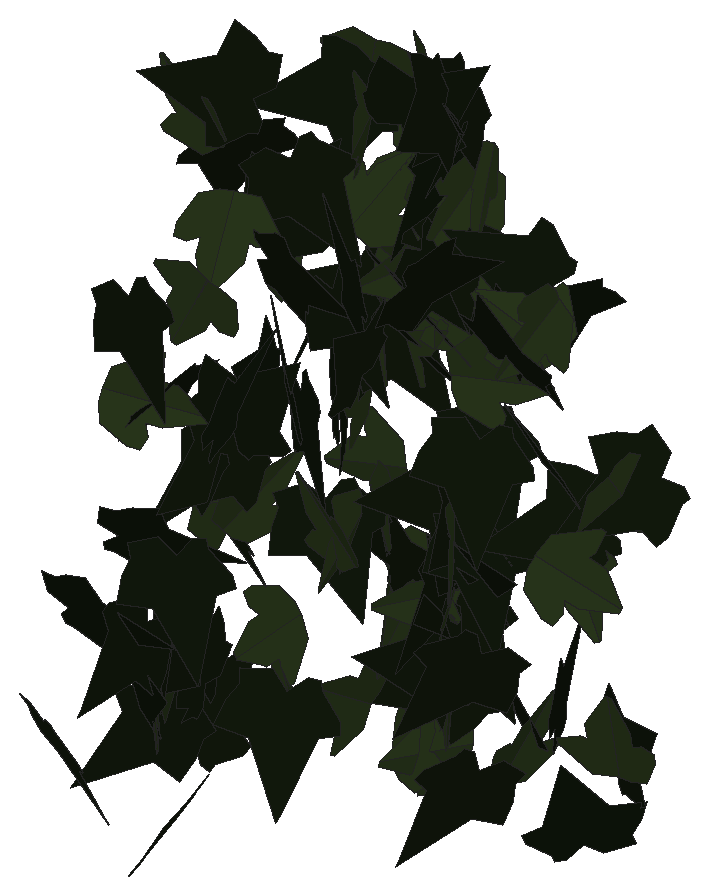
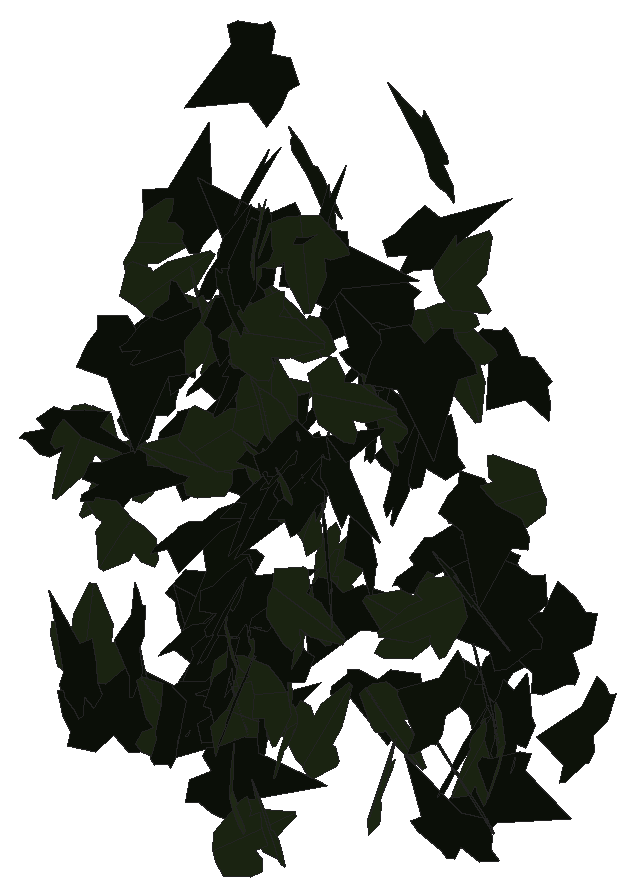
# SketchUp Ruby script. Lengths in inches.
U = 1.inch
M = Sketchup.active_model
def pt(a) = Geom::Point3d.new(a.map { |v| v * U })
def face(e, loops, mat)
  f = e.add_face(loops[0].map { |a| pt(a) })
  loops[1..].each { |l| e.add_face(l.map { |a| pt(a) }).erase! }
  f.material = f.back_material = mat if mat
  f
end
# faces: each face lists its corners as indices into pts; further lists are holes
def faces(e, pts, list, mat = nil) = list.each { |f| face(e, (f[0].is_a?(Array) ? f : [f]).map { |l| l.map { |i| pts[i] } }, mat) }
# xy, xz, yz: faces in a plane at the given z, y or x. An outline is a flat list of corners, or four numbers for a rectangle; further outlines are holes
def ring(l) = l.size == 4 ? [[l[0], l[1]], [l[2], l[1]], [l[2], l[3]], [l[0], l[3]]] : l.each_slice(2).to_a
def flat(e, list, mat, &to3) = list.each { |f| face(e, (f[0].is_a?(Array) ? f : [f]).map { |l| ring(l).map { |u, v| to3.(u, v) } }, mat) }
def xy(e, z, list, mat = nil) = flat(e, list, mat) { |x, y| [x, y, z] }
def xz(e, y, list, mat = nil) = flat(e, list, mat) { |x, z| [x, y, z] }
def yz(e, x, list, mat = nil) = flat(e, list, mat) { |y, z| [x, y, z] }
def lines(e, pts, list) = list.each { |a, b| e.add_line(pt(pts[a]), pt(pts[b])) }
# prism: a flat outline (further loops are holes) pulled along v
def prism(e, loops, v, mat = nil)
  f = face(e, loops, mat); d = Geom::Vector3d.new(v.map { |x| x * U })
  f.pushpull(f.normal.samedirection?(d) ? d.length : -d.length)
end
def box(e, o, s, mat = nil) = prism(e, [[o, [o[0] + s[0], o[1], o[2]], [o[0] + s[0], o[1] + s[1], o[2]], [o[0], o[1] + s[1], o[2]]]], [0, 0, s[2]], mat)
def at(x, y, z, deg = 0) = Geom::Transformation.translation(pt([x, y, z])) * Geom::Transformation.rotation(ORIGIN, Z_AXIS, deg.degrees)
def axes(o, x, y, z) = Geom::Transformation.new([*x, 0, *y, 0, *z, 0, *pt(o).to_a, 1])
def part(name) = M.definitions.add(name)
# library, detail: a bought-in or finely detailed component or shape, given as its bounding box
def library(name, o, s) = part(name).tap { |d| box(d.entities, o, s) }
def detail(e, o, s) = box(e.add_group.entities, o, s)
def put(e, d, t, mat = nil) = e.add_instance(d, t).tap { |i| i.material = mat if mat }
def group(e, t, mat = nil) = e.add_group.tap { |g| g.transformation = t; g.material = mat if mat }.entities
root = M.entities
M.materials.add("efeu1").color = [18, 25, 13]
M.materials.add("efeu2").color = [43, 57, 29]
c1 = part("ivyleaf_9")
p = [[1.54,2.16,1.25],[1.36,2.04,1.19],[-0.21,0.99,0.68],[-0.71,1.11,0.82],[-0.85,0.86,0.67],[-0.8,0.17,0.21],
  [-0.9,-0.01,0.1],[-0.67,-0.16,-0.02],[-0.08,-0.08,-0.05],[-0.03,-0.6,-0.4],[0.65,-0.88,-0.66],[0.83,-0.6,-0.49],
  [1.29,-0.42,-0.43],[1.8125,-0.07,-0.26],[1.21,0.44,0.15]]
faces(c1.entities,p,[[0,1,2,3,4,5,6,7,8,9,10,11,12,13,14]],"efeu1")
c2 = part("ivyleaf_10")
p = [[0,0.5,-0.03],[-0.0625,2.02,-0.43],[-0.19,2.01,-0.46],[-0.54,1.05,-0.29],[-0.52,0.625,-0.18],[-0.83,0.76,-0.28],
  [-1.16,0.64,-0.33],[-1.15,0.33,-0.24],[-0.77,-0.39,0.02],[-0.3,-0.51,0.16],[0.04,-0.48,0.23],[-0.02,2.01,-0.4375],
  [-0.06,2.01,-0.43],[0.04,-0.49,0.23],[0.67,-0.49,0.14],[1.38,0.36,-0.2],[1.375,0.51,-0.24],[0.81,0.65,-0.19],
  [0.62,0.59,-0.15],[0.6,1.09,-0.28],[0.5,1.23,-0.31]]
faces(c2.entities,p,[[0,1,2,3,4,5,6,7,8,9,10],[11,12,0,13,14,15,16,17,18,19,20]],"efeu2")
put(root,c1,axes([47.99,215.16,220.86],[-0.17169,0.44086,0.16175],[0.0482,-0.15477,0.47299],[0.46712,0.17801,0.01065]))
put(root,c1,axes([46.04,216.63,214.23],[-0.07459,0.45103,0.20252],[-0.03957,0.1987,-0.45711],[-0.49282,-0.08422,0.00606]))
put(root,c1,axes([43.89,217.16,214.625],[0.30514,-0.33363,0.2135],[0.14379,-0.15781,-0.45213],[0.36907,0.33732,-0.00036]))
put(root,c1,axes([48.8,216.82,221.22],[-0.16626,0.34154,0.32513],[-0.13737,0.29472,-0.37983],[-0.4511,-0.21563,-0.00417]))
put(root,c1,axes([49.54,216.83,222.625],[-0.06882,0.21369,-0.44676],[-0.12086,0.43017,0.22438],[0.48027,0.13888,-0.00756]))
put(root,c1,axes([44.74,217.89,215.97],[0.05227,-0.05863,-0.49379],[0.24772,-0.42744,0.07698],[-0.43116,-0.25269,-0.01564]))
put(root,c1,axes([43.93,217.58,216.05],[0.28747,-0.12982,0.38796],[0.36207,-0.13998,-0.31513],[0.19043,0.46212,0.01353]))
put(root,c1,axes([49.72,217.85,217.31],[0.00747,0.18447,-0.46467],[-0.07922,-0.45841,-0.18326],[-0.49363,0.07636,0.02238]))
put(root,c1,axes([45.33,217.75,217.09],[-0.26087,-0.25582,-0.34133],[0.23496,0.24775,-0.36526],[0.35601,-0.35096,-0.00905]))
put(root,c1,axes([44.6,217.78,220.27],[-0.21419,-0.0866,-0.44342],[0.40773,0.17435,-0.231],[0.19463,-0.46055,-0.00407]))
put(root,c1,axes([49.43,218.17,215.51],[-0.02735,0.20302,-0.45611],[0.02463,-0.45569,-0.20431],[-0.49864,-0.03364,0.01493]))
put(root,c1,axes([44.26,218.28,214.91],[0.06762,-0.11488,0.4819],[0.22476,-0.42632,-0.13317],[0.44149,0.23463,-0.00601]))
put(root,c1,axes([47.65,218.22,221.05],[0.10012,-0.38158,0.3072],[-0.02038,0.31004,0.39174],[-0.48945,-0.09096,0.04653]))
put(root,c2,axes([45.28,218.3,220.42],[-0.42148,-0.06864,0.26009],[-0.25219,-0.06735,-0.42645],[0.09358,-0.49066,0.02216]))
put(root,c2,axes([44.33,218.53,214.92],[-0.15127,0.27122,-0.39186],[0.1831,-0.3465,-0.3105],[-0.43999,-0.23744,0.00551]))
put(root,c1,axes([44.46,218.74,214.35],[-0.02016,0.00124,-0.49959],[0.01647,-0.49973,-0.0019],[-0.49932,-0.01653,0.02011]))
put(root,c1,axes([44.12,218.28,216.77],[0.35731,-0.00643,0.3497],[0.34938,0.02964,-0.35644],[-0.01615,0.49908,0.02567]))
put(root,c1,axes([46.25,218.625,215.23],[-0.29745,-0.33879,-0.2162],[0.14429,0.16101,-0.45084],[0.3751,-0.3306,0.00198]))
put(root,c1,axes([45.59,218.51,218.67],[-0.16318,0.01348,0.47243],[0.40966,-0.2452,0.1485],[0.23569,0.43554,0.06898]))
put(root,c1,axes([49.5,218.69,220.84],[0.43274,-0.21487,0.12871],[-0.1132,0.0614,0.48313],[-0.22343,-0.44728,0.0045]))
put(root,c2,axes([44.12,218.29,218.62],[0.09254,0.11107,0.47864],[0.27138,0.39448,-0.14401],[-0.40962,0.28644,0.01272]))
put(root,c1,axes([44.42,218.78,216.05],[-0.20659,-0.00926,-0.45523],[0.44787,-0.09422,-0.20134],[-0.08205,-0.49096,0.04722]))
put(root,c1,axes([46.41,218.61,218.98],[0.03367,-0.24189,0.4363],[-0.08064,0.4289,0.24401],[-0.4923,-0.0868,-0.01013]))
put(root,c2,axes([45.16,218.91,221.15],[0.36505,0.32327,-0.11059],[-0.0819,-0.07433,-0.48761],[-0.33171,0.37413,-0.00131]))
put(root,c1,axes([45.8,218.9375,220.72],[0.2344,0.04973,-0.43884],[0.42362,0.11519,0.23932],[0.12491,-0.484,0.01187]))
put(root,c1,axes([44.37,218.63,218.53],[0.02948,0.49035,0.09323],[0.00081,0.09335,-0.49121],[-0.49913,0.02911,0.00471]))
put(root,c1,axes([44.97,219.4,217.79],[-0.18945,-0.33461,0.3196],[-0.16866,-0.27166,-0.38439],[0.43089,-0.25345,-0.00994]))
put(root,c1,axes([44.76,219.12,217.71],[-0.46066,0.16849,-0.09697],[0.08681,-0.04487,-0.49036],[-0.17394,-0.46861,0.01209]))
put(root,c1,axes([44.34,219.44,215],[-0.02739,-0.2858,0.40935],[-0.0486,-0.40649,-0.28706],[0.49688,-0.05552,-0.00551]))
put(root,c2,axes([44.49,218.7,214.85],[-0.00152,-0.08865,-0.49208],[-0.04087,0.49045,-0.08823],[0.49832,0.03995,-0.00874]))
put(root,c2,axes([44.68,219.07,222.01],[-0.38714,0.10727,-0.29769],[-0.28541,0.08472,0.4017],[0.13662,0.48095,-0.00437]))
put(root,c1,axes([45.35,219.42,218.61],[-0.03353,0.0613,0.49509],[-0.10617,-0.48572,0.05295],[0.48745,-0.10157,0.04559]))
put(root,c1,axes([45.05,219.43,222.43],[-0.15128,0.00179,0.47656],[-0.39667,-0.2776,-0.12488],[0.26414,-0.41586,0.08541]))
put(root,c2,axes([49.49,219.46,221.06],[0.0773,0.22623,-0.43914],[-0.11682,-0.4235,-0.23874],[-0.47998,0.13951,-0.01262]))
put(root,c1,axes([46.31,219.43,218.86],[-0.0575,0.149,0.47381],[0.07117,-0.46958,0.1563],[0.49156,0.08542,0.03279]))
put(root,c1,axes([44.69,219.04,214.7],[-0.2061,0.29988,0.34292],[-0.19811,0.27993,-0.36386],[-0.41022,-0.28585,0.00343]))
put(root,c2,axes([46.54,219.27,217.01],[-0.35888,0.19083,-0.29118],[-0.27946,0.09148,0.40439],[0.20762,0.453,0.041]))
put(root,c1,axes([48.37,219.55,218.92],[-0.14024,-0.46394,-0.12286],[0.04991,0.1132,-0.48445],[0.47733,-0.14815,0.01456]))
put(root,c1,axes([44.375,219.3,213.77],[-0.28637,0.15636,0.37887],[0.33335,-0.18007,0.32627],[0.23848,0.43946,-0.00111]))
put(root,c2,axes([44.75,219.1,217.11],[-0.03995,-0.08244,-0.49154],[0.27053,0.41056,-0.09085],[0.41859,-0.2732,0.0118]))
put(root,c2,axes([46.43,219.84,214.7],[-0.05422,-0.25576,-0.4262],[-0.10347,-0.41353,0.26132],[-0.48616,0.11653,-0.00808]))
put(root,c2,axes([45.51,219.52,215.57],[0.3507,-0.14006,-0.32771],[-0.31087,0.10461,-0.37738],[0.17428,0.46844,-0.01371]))
put(root,c2,axes([46.23,219.89,216.98],[0.06099,-0.17211,0.46547],[0.21407,-0.41397,-0.18112],[0.44772,0.22138,0.02319]))
put(root,c1,axes([45.6875,219.46,221.76],[-0.1147,-0.20196,-0.44278],[0.21685,0.38605,-0.23226],[0.43568,-0.24531,-0.00097]))
put(root,c2,axes([49.13,219.76,220.46],[0.18596,0.30213,0.35233],[-0.20413,-0.28764,0.35439],[0.41683,-0.27565,0.01637]))
put(root,c1,axes([46.16,219.65,220.1],[0.22341,-0.41117,-0.17616],[-0.05671,0.16928,-0.46704],[0.4437,0.22866,0.029]))
put(root,c2,axes([44.96,219.41,216.84],[-0.0438,-0.33988,0.36409],[0.03814,0.36213,0.34265],[-0.49662,0.05779,-0.0058]))
put(root,c1,axes([48.92,219.9375,218.91],[0.40702,-0.15845,-0.24337],[0.2273,-0.08699,0.43677],[-0.18076,-0.46618,0.00122]))
put(root,c1,axes([45.46,219.92,218.35],[-0.1148,0.01134,-0.48651],[0.48636,-0.01439,-0.1151],[-0.01662,-0.49966,-0.00772]))
put(root,c1,axes([45.26,219.72,220.66],[-0.25055,0.15868,0.40255],[0.34038,-0.21491,0.29657],[0.26714,0.42265,-0.00034]))
put(root,c2,axes([49.52,219.5,217.7],[0.12167,0.28036,0.39572],[0.14907,0.36661,-0.30557],[-0.46149,0.19234,0.00563]))
put(root,c1,axes([45.91,219.81,217.15],[-0.18585,-0.3015,-0.35293],[0.1696,0.30978,-0.35394],[0.43208,-0.25127,-0.01287]))
put(root,c1,axes([49.61,219.95,213.91],[0.3522,0.14995,0.32167],[-0.29593,-0.12609,0.38279],[0.19591,-0.46002,-0.00007]))
put(root,c2,axes([45.31,219.84,214.26],[-0.26282,0.42147,-0.05736],[-0.03543,0.0455,0.49666],[0.42388,0.26513,0.00595]))
put(root,c1,axes([47.23,220.3125,222.67],[-0.04162,-0.23336,0.44024],[-0.06095,-0.43607,-0.23691],[0.49452,-0.07339,0.00786]))
put(root,c2,axes([46.13,220.22,222.125],[-0.07635,0.06216,0.49021],[0.33725,-0.35598,0.09767],[0.36115,0.34556,0.01243]))
put(root,c1,axes([48.32,220.09,220.36],[0.08806,0.0112,-0.49206],[0.48948,0.05033,0.08874],[0.05152,-0.49733,-0.0021]))
put(root,c1,axes([43.93,220.2,216.26],[0.22128,-0.33793,0.29468],[0.19915,-0.22035,-0.40223],[0.40172,0.29538,0.03708]))
put(root,c2,axes([45.25,219.86,220.04],[0.22068,0.00089,0.44867],[-0.43181,0.13621,0.21211],[-0.12185,-0.48109,0.06088]))
put(root,c2,axes([46.03,220.43,218.46],[-0.00525,-0.19823,-0.45899],[0.02373,-0.4586,0.19779],[-0.49941,-0.01971,0.01423]))
put(root,c2,axes([49.91,220.16,214.96],[-0.48711,-0.11174,-0.0153],[-0.01208,-0.01575,0.49961],[-0.11213,0.4871,0.01265]))
put(root,c1,axes([44.43,219.96,221.44],[0.13293,0.4408,-0.19501],[-0.06511,-0.18401,-0.46033],[-0.47759,0.14778,0.00848]))
put(root,c1,axes([49.42,220.41,217.86],[-0.30264,-0.14157,0.37198],[-0.31304,-0.20391,-0.3323],[0.24579,-0.43403,0.03479]))
put(root,c1,axes([45.96,220.46,222.43],[-0.10597,-0.16668,-0.45933],[-0.21301,-0.40725,0.19692],[-0.43977,0.23742,0.0153]))
put(root,c2,axes([46.19,220.16,220.98],[0.41876,-0.00156,-0.27319],[0.27284,0.02802,0.41806],[0.01401,-0.49921,0.02432]))
put(root,c2,axes([48.42,220.14,214.4],[0.03137,-0.45907,0.19564],[0.01505,0.1968,0.45939],[-0.49879,-0.02293,0.02617]))
put(root,c2,axes([46.08,220.5,219.41],[0.16434,-0.08747,0.46405],[0.39857,-0.23781,-0.18598],[0.25325,0.43104,-0.00844]))
put(root,c2,axes([46.08,220.54,217],[-0.06596,0.08423,-0.48842],[0.2724,-0.40548,-0.10671],[-0.41407,-0.28016,0.0076]))
put(root,c1,axes([49.16,220,215.32],[-0.00316,-0.01195,0.49985],[0.05719,0.49657,0.01224],[-0.49671,0.05725,-0.00177]))
put(root,c2,axes([49.0625,220.34,217.31],[0.41107,0.06457,0.27722],[0.27293,0.04886,-0.41608],[-0.08082,0.4934,0.00493]))
put(root,c1,axes([47.04,220.2,220.6875],[0.22053,-0.26657,-0.36098],[-0.20999,0.29415,-0.34551],[0.39658,0.30399,0.01778]))
put(root,c1,axes([47.14,220.72,214.99],[-0.10074,-0.06541,0.48536],[-0.38447,-0.29638,-0.11974],[0.30337,-0.39734,0.00942]))
put(root,c1,axes([49.63,220.57,214.75],[-0.03926,0.05589,0.49531],[0.23831,-0.43428,0.0679],[0.4378,0.24141,0.00746]))
put(root,c1,axes([50.08,220.6875,218.56],[-0.39718,-0.21572,0.21381],[-0.18545,-0.10651,-0.45196],[0.24054,-0.43832,0.00459]))
put(root,c2,axes([46.15,220.7,215.5],[-0.06394,0.22506,-0.44188],[0.11459,-0.42677,-0.23395],[-0.48247,-0.13118,0.00299]))
put(root,c2,axes([49.79,220.29,218.54],[-0.11537,-0.4057,-0.26851],[0.12094,0.24338,-0.41969],[0.47123,-0.16179,0.04197]))
put(root,c1,axes([45.87,220.22,218.29],[-0.01475,0.026,-0.49911],[-0.47799,0.1451,0.02169],[0.14596,0.47778,0.02057]))
put(root,c1,axes([46.57,220.43,222.2],[-0.08827,-0.03346,0.49101],[0.47563,-0.13396,0.07637],[0.12644,0.48056,0.05548]))
put(root,c2,axes([46.625,220.8125,220.21],[0.01833,0.05294,-0.49685],[-0.2625,-0.42203,-0.05465],[-0.42515,0.26285,0.01232]))
put(root,c1,axes([47.92,220.76,214.81],[0.12597,-0.20474,0.43842],[0.20489,-0.38785,-0.23999],[0.43835,0.24012,-0.01382]))
put(root,c2,axes([47,220.78,216.75],[0.11568,-0.1584,0.45992],[0.35126,-0.29983,-0.19162],[0.3365,0.36744,0.04191]))
put(root,c1,axes([46.27,220.59,216.125],[0.13482,-0.07658,0.47535],[0.39173,-0.26956,-0.15453],[0.27994,0.41409,-0.01269]))
put(root,c1,axes([45.4,220.65,219.66],[-0.33353,0.21174,-0.30647],[0.24964,-0.17826,-0.39485],[-0.27647,-0.4164,0.01319]))
put(root,c2,axes([46.97,220.85,215.9],[0.00955,0.00971,-0.49981],[-0.33517,-0.37078,-0.01361],[-0.37091,0.3353,-0.00057]))
put(root,c2,axes([46.19,220.61,220.14],[0.08457,-0.04494,0.49074],[0.49259,0.02204,-0.08287],[-0.01419,0.49749,0.04801]))
put(root,c2,axes([45.49,220.64,220.61],[0.06519,0.04156,0.49399],[-0.46192,-0.17576,0.07575],[0.17994,-0.46624,0.01547]))
put(root,c2,axes([46.5,220.87,222.52],[-0.08254,0.04965,0.49063],[0.37038,-0.32219,0.09491],[0.32558,0.37911,0.0164]))
put(root,c1,axes([48.35,220.86,220.47],[-0.15797,-0.4433,-0.1689],[-0.02027,-0.17155,0.46921],[-0.47396,0.15509,0.03623]))
put(root,c1,axes([45.99,220.89,219.42],[-0.09816,-0.05118,0.48759],[-0.4378,-0.21467,-0.11067],[0.22067,-0.44866,-0.00267]))
put(root,c1,axes([46.91,220.92,216.1875],[-0.05551,0.04258,-0.49508],[0.30101,-0.39348,-0.06759],[-0.39536,-0.30555,0.01805]))
put(root,c2,axes([46,220.6,222.84],[-0.45945,-0.1506,0.12738],[-0.12207,-0.03655,-0.48349],[0.15494,-0.47538,-0.00318]))
put(root,c1,axes([46.88,220.87,221.74],[-0.0987,0.16348,-0.46209],[0.25011,-0.38859,-0.1909],[-0.42155,-0.26883,-0.00507]))
put(root,c2,axes([46.47,220.625,213.61],[0.45413,-0.20026,-0.06054],[0.05824,-0.01796,0.49627],[-0.20094,-0.45779,0.00701]))
put(root,c1,axes([46.1,220.71,219.85],[0.39094,-0.24838,0.18833],[0.1577,-0.10298,-0.46317],[0.26888,0.42155,-0.00218]))
put(root,c2,axes([46.18,220.68,217.39],[-0.11108,-0.00936,0.48742],[-0.47632,-0.10439,-0.11055],[0.10383,-0.48889,0.01428]))
put(root,c1,axes([47.1,220.5625,217.63],[0.46194,-0.11956,-0.1494],[-0.14423,0.03897,-0.47716],[0.12574,0.48393,0.00152]))
put(root,c2,axes([46.9375,220.81,215.94],[0.31425,-0.37755,0.0933],[0.05923,-0.07209,-0.49122],[0.38437,0.31978,-0.00058]))
put(root,c2,axes([46.47,221.01,221.37],[-0.0454,-0.11815,0.48372],[-0.17932,-0.44925,-0.12656],[0.46452,-0.18497,-0.00158]))
put(root,c1,axes([46.92,221.08,222.43],[0.12632,-0.15955,-0.45671],[0.30002,-0.34446,0.20332],[-0.37952,-0.32541,0.00871]))
put(root,c2,axes([46.76,221.05,213.68],[-0.01506,0.08922,0.49174],[-0.02389,-0.49153,0.08845],[0.4992,-0.02083,0.01906]))
put(root,c1,axes([46.93,221.07,217.125],[-0.14546,-0.1427,0.45659],[-0.34864,-0.29515,-0.20331],[0.32755,-0.37753,-0.01363]))
put(root,c1,axes([47.01,220.82,216.26],[0.39742,-0.00338,-0.30339],[0.30162,0.05868,0.39444],[0.03294,-0.49653,0.04868]))
put(root,c1,axes([47.3,220.9,216.73],[0.01002,-0.49448,-0.07341],[0.04791,0.07404,-0.49216],[0.4976,0.00282,0.04886]))
put(root,c1,axes([46.48,220.93,222.38],[0.32938,-0.0627,-0.37091],[0.36859,-0.0447,0.33488],[-0.07516,-0.49403,0.01678]))
put(root,c1,axes([46.73,221.125,215.65],[-0.03315,-0.16956,0.4692],[-0.03952,-0.46787,-0.17187],[0.49733,-0.04848,0.01762]))
put(root,c2,axes([46.7,220.99,215.66],[0.16463,0.25714,-0.39595],[-0.21319,-0.33366,-0.30533],[-0.42125,0.26935,-0.00022]))
put(root,c2,axes([46.8,220.91,221.27],[0.14793,0.39054,-0.27494],[-0.09461,-0.25817,-0.41761],[-0.46815,0.17558,-0.00248]))
put(root,c1,axes([46.01,220.46,219.27],[0.08495,-0.10477,-0.48146],[-0.17489,0.45034,-0.12886],[0.46065,0.1903,0.03986]))
put(root,c1,axes([47.39,220.89,218.1875],[0.00965,-0.48048,-0.13802],[0.04623,0.13832,-0.47826],[0.49777,-0.00353,0.04709]))
put(root,c2,axes([46.12,220.9,219.09],[0.15845,-0.10085,-0.46338],[0.4038,-0.2275,0.18759],[-0.24867,-0.43367,0.00935]))
put(root,c2,axes([46.36,220.84,220.34],[0.47204,-0.16042,0.03796],[0.03823,-0.00547,-0.49851],[0.16036,0.47353,0.0071]))
put(root,c1,axes([45.78,220.71,219.33],[0.46495,-0.12133,0.13819],[0.13339,-0.03614,-0.48052],[0.12659,0.48371,-0.00124]))
put(root,c1,axes([46.86,220.96,220.9],[0.05189,-0.49455,-0.05223],[-0.00361,0.05214,-0.49726],[0.49729,0.05198,0.00184]))
put(root,c2,axes([47.36,220.66,218.94],[-0.05724,-0.0359,0.49541],[0.43081,0.24464,0.0675],[-0.24725,0.43458,0.00292]))
put(root,c1,axes([46.93,221.19,216.84],[-0.02235,-0.3009,0.39869],[-0.04572,-0.39619,-0.30157],[0.4974,-0.04993,-0.0098]))
put(root,c1,axes([46.16,220.71,219.26],[0.13503,-0.35137,-0.3291],[-0.07292,0.32293,-0.3747],[0.47587,0.14919,0.03597]))
put(root,c2,axes([46.23,220.9,216.0625],[-0.23264,0.03424,-0.44126],[0.40119,-0.19419,-0.22658],[-0.18689,-0.45948,0.06288]))
put(root,c1,axes([46.96,221.12,214.73],[-0.09491,-0.15302,-0.46645],[-0.13012,-0.45026,0.17418],[-0.47335,0.15445,0.04564]))
put(root,c1,axes([46.95,220.93,222.01],[-0.38224,0.21302,-0.24189],[0.20877,-0.12225,-0.43757],[-0.24557,-0.43552,0.00451]))
put(root,c2,axes([47.16,221,219.49],[0.19287,0.25749,0.38275],[-0.22591,-0.30898,0.32171],[0.4022,-0.29703,-0.00285]))
put(root,c2,axes([47.12,221.07,221.3125],[0.10497,0.31869,-0.3707],[-0.17474,-0.32964,-0.33287],[-0.45656,0.19944,0.04217]))
put(root,c1,axes([48.61,220.67,220.4],[0.15589,0.45792,-0.12651],[-0.03854,-0.12052,-0.48372],[-0.47351,0.16057,-0.00229]))
put(root,c2,axes([46.66,221.125,214.51],[0.12754,-0.10065,0.47287],[0.36612,-0.29928,-0.16245],[0.31574,0.38769,-0.00264]))
put(root,c2,axes([47.31,221,221.63],[0.39733,-0.26011,0.15644],[0.1287,-0.08902,-0.47488],[0.27489,0.41764,-0.00379]))
put(root,c1,axes([46.98,220.87,215.64],[-0.14277,-0.19159,-0.43921],[0.31074,0.31185,-0.23704],[0.36477,-0.34065,0.03002]))
